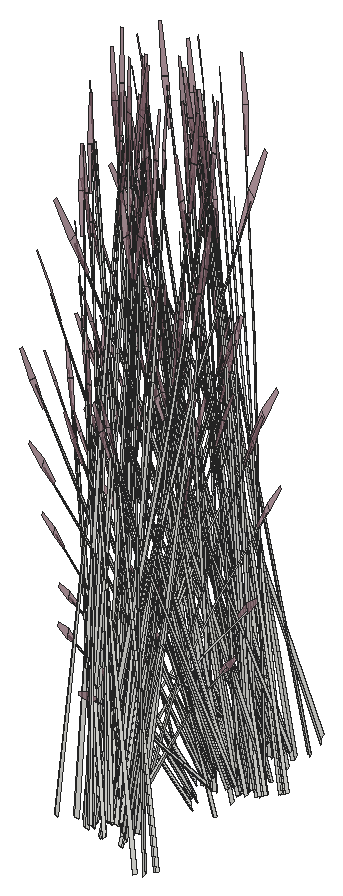
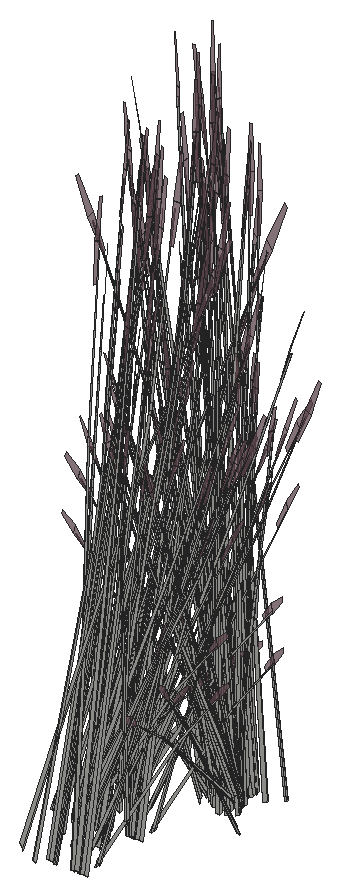
# SketchUp Ruby script. Lengths in inches.
U = 1.inch
M = Sketchup.active_model
def pt(a) = Geom::Point3d.new(a.map { |v| v * U })
def face(e, loops, mat)
  f = e.add_face(loops[0].map { |a| pt(a) })
  loops[1..].each { |l| e.add_face(l.map { |a| pt(a) }).erase! }
  f.material = f.back_material = mat if mat
  f
end
# faces: each face lists its corners as indices into pts; further lists are holes
def faces(e, pts, list, mat = nil) = list.each { |f| face(e, (f[0].is_a?(Array) ? f : [f]).map { |l| l.map { |i| pts[i] } }, mat) }
# xy, xz, yz: faces in a plane at the given z, y or x. An outline is a flat list of corners, or four numbers for a rectangle; further outlines are holes
def ring(l) = l.size == 4 ? [[l[0], l[1]], [l[2], l[1]], [l[2], l[3]], [l[0], l[3]]] : l.each_slice(2).to_a
def flat(e, list, mat, &to3) = list.each { |f| face(e, (f[0].is_a?(Array) ? f : [f]).map { |l| ring(l).map { |u, v| to3.(u, v) } }, mat) }
def xy(e, z, list, mat = nil) = flat(e, list, mat) { |x, y| [x, y, z] }
def xz(e, y, list, mat = nil) = flat(e, list, mat) { |x, z| [x, y, z] }
def yz(e, x, list, mat = nil) = flat(e, list, mat) { |y, z| [x, y, z] }
def lines(e, pts, list) = list.each { |a, b| e.add_line(pt(pts[a]), pt(pts[b])) }
# prism: a flat outline (further loops are holes) pulled along v
def prism(e, loops, v, mat = nil)
  f = face(e, loops, mat); d = Geom::Vector3d.new(v.map { |x| x * U })
  f.pushpull(f.normal.samedirection?(d) ? d.length : -d.length)
end
def box(e, o, s, mat = nil) = prism(e, [[o, [o[0] + s[0], o[1], o[2]], [o[0] + s[0], o[1] + s[1], o[2]], [o[0], o[1] + s[1], o[2]]]], [0, 0, s[2]], mat)
def at(x, y, z, deg = 0) = Geom::Transformation.translation(pt([x, y, z])) * Geom::Transformation.rotation(ORIGIN, Z_AXIS, deg.degrees)
def axes(o, x, y, z) = Geom::Transformation.new([*x, 0, *y, 0, *z, 0, *pt(o).to_a, 1])
def part(name) = M.definitions.add(name)
# library, detail: a bought-in or finely detailed component or shape, given as its bounding box
def library(name, o, s) = part(name).tap { |d| box(d.entities, o, s) }
def detail(e, o, s) = box(e.add_group.entities, o, s)
def put(e, d, t, mat = nil) = e.add_instance(d, t).tap { |i| i.material = mat if mat }
def group(e, t, mat = nil) = e.add_group.tap { |g| g.transformation = t; g.material = mat if mat }.entities
root = M.entities
M.materials.add("LightPink_Translucent").color = [144, 107, 117]
M.materials["LightPink_Translucent"].alpha = 0.75
c1 = part("blade")
p = [[2.15,0.21,22],[0,0.17,0],[0.09,0.45,0],[2.18,0.31,22],[2.29,0.31,22],[0.38,0.45,0],
  [2.48,0.24,33],[2.49,0.24,33],[2.48,0.22,33]]
faces(c1.entities,p,[[0,1,2,3],[4,5,2,3],[6,3,4,7],[8,0,3,6]])
c2 = part("seeds")
p = [[0.3,-0.1,1.38],[-0.01,-0.03,1.59],[-0.01,-0.03,0.03],[0.14,-0.07,-0.07],[0.29,-0.03,3],[0.15,0.01,3.11]]
faces(c2.entities,p,[[0,1,2,3],[1,0,4,5]],"LightPink_Translucent")
c3 = part("blade with seeds")
put(c3.entities,c1,at(0,0,0))
put(c3.entities,c2,axes([2.4,0.25,30.99],[1.5799,-0.05474,1.17369],[-0.12525,1.92788,0.29478],[-0.07173,-0.02425,1.56792]))
put(root,c3,axes([289.25,449.71,5.65],[0.78943,0.17416,-0.06488],[-0.24284,0.53604,-0.29416],[-0.12912,0.08139,0.97024]))
put(root,c3,axes([294.85,448.71,2.06],[-0.60257,0.49041,-0.62353],[-0.74854,-0.44469,-0.16365],[-0.24146,0.12234,1.37633]))
put(root,c3,axes([286.96,451.98,2.36],[-0.74176,0.59212,0.45755],[-0.88124,-0.52269,0.17955],[0.17882,-0.05909,1.58856]))
put(root,c3,axes([295.84,450.05,2.02],[-0.83726,0.32623,-0.49651],[-0.50045,-0.58498,0],[-0.19069,0.0743,1.57504]))
put(root,c3,axes([285.68,451.01,2.47],[-0.25843,0.64844,0.17642],[-0.9457,-0.1835,0.35086],[0.16336,-0.00316,1.60407]))
put(root,c3,axes([287.65,451.73,2.62],[0.17258,-0.58229,0.1448],[0.84319,0.10108,-0.41347],[0.15345,0.05979,1.26744]))
put(root,c3,axes([290.61,448.14,5.03],[0.82753,0.35977,-0.1216],[-0.47675,0.52101,-0.67495],[-0.2338,0.18111,1.02557]))
put(root,c3,axes([287.29,451.88,2.72],[-0.53742,-0.54764,0.44739],[0.81403,-0.38564,-0.21531],[0.17391,0.06776,1.43643]))
put(root,c3,axes([291.02,448.57,4.68],[0.22982,0.59576,-0.51099],[-0.87033,0.10422,-0.3958],[-0.24941,0.16002,0.97773]))
put(root,c3,axes([292.07,449.26,5.05],[0.60531,-0.34352,0.35414],[0.573,0.39225,-0.4572],[-0.08718,0.19929,0.87481]))
put(root,c3,axes([287.57,451.92,2.67],[0.90324,-0.43318,-0.29095],[0.60064,0.61207,-0.50002],[0.22285,0.06216,1.59708]))
put(root,c3,axes([296.125,447.36,2.84],[-0.02444,-0.61432,1.41272],[1.10603,0.15924,0.59816],[-0.26159,0.33615,1.3335]))
put(root,c3,axes([291.52,449.57,4.73],[-0.73517,-0.0304,0.0643],[0.02016,-0.45906,0.50621],[-0.07693,0.17585,0.77189]))
put(root,c3,axes([291.75,449.61,4.73],[-0.63704,-0.44518,0.48003],[0.67652,-0.38394,0.3958],[-0.11751,0.20886,0.9933]))
put(root,c3,axes([288.25,452.625,2.21],[1.00089,0,0],[0,0.67548,0],[0,0,1.78407]))
put(root,c3,axes([288.54,451.04,2.47],[-0.96132,0.17317,0.17642],[-0.23737,-0.64447,0.35086],[0.08574,0.0939,1.60407]))
put(root,c3,axes([289.61,451.01,2.03],[0.21015,0.56852,-0.30978],[-0.83462,0.16144,0.30978],[0.16826,0.06556,1.38974]))
put(root,c3,axes([287.93,452.28,2.38],[-1.13071,-0.13747,0.49198],[0.23011,-0.77639,0.19306],[0.16524,0.07497,1.70813]))
put(root,c3,axes([287.03,454.2,2.2],[-0.29189,-0.56252,0],[0.83351,-0.19699,0],[0,0,1.54371]))
put(root,c3,axes([291.56,448.48,3.875],[0.16657,-0.22426,1.71376],[0.69879,0.4641,0.13857],[-0.31524,0.28926,0.73262]))
put(root,c3,axes([288.12,454.12,2.18],[0.93921,-0.22138,-0.19198],[0.33003,0.6377,0.00008],[0.10367,-0.02447,1.73897]))
put(root,c3,axes([288.23,452.91,2.21],[0.62448,0.42144,0],[-0.62448,0.42144,0],[0,0,1.69266]))
put(root,c3,axes([289.92,452.73,2.47],[-0.70288,-0.47526,0.17642],[0.70832,-0.46097,0.35086],[-0.07763,0.09706,1.60407]))
put(root,c3,axes([291.75,449.74,4.53],[-0.60531,0.34352,-0.35414],[-0.573,-0.39225,0.4572],[-0.08718,0.19929,0.87481]))
put(root,c3,axes([289.66,449.64,4.72],[-0.02224,0.12912,1.74944],[0.63107,0.44917,-0.27667],[-0.16521,0.21241,0.14031]))
put(root,c3,axes([291.68,449.35,5.4],[0.98321,0.03233,-0.13498],[-0.02687,0.61208,-0.74919],[-0.0683,0.23574,1.13838]))
put(root,c3,axes([292.52,459.42,3.875],[0.2045,0.20949,1.71376],[-0.94495,0.17636,0.13857],[-0.21357,-0.32887,0.73262]))
put(root,c3,axes([292.14,451.08,2.77],[-0.02315,-0.38796,1.1486],[0.57853,0.27671,0.84392],[-0.11378,0.18492,0.25299]))
put(root,c3,axes([294.08,458.03,4.72],[-0.13683,-0.09148,1.74944],[-0.91315,0.058,-0.27667],[-0.14574,-0.2188,0.14031]))
put(root,c3,axes([288.22,452.42,2.72],[0.43405,-0.58792,0.44739],[0.90188,0.28295,-0.21531],[0,0.13553,1.43643]))
put(root,c3,axes([295.04,459.58,4.98],[-0.42698,-0.53052,-0.71045],[0.87893,-0.29566,0.08574],[-0.09984,-0.25633,1.00501]))
put(root,c3,axes([292.27,458.87,2.59],[-0.05417,0.21344,1.43002],[-0.79196,0.17867,-0.30754],[-0.18512,-0.27588,0.61141]))
put(root,c3,axes([288.06,452.76,2.29],[0,0.75458,-0.05637],[-1.11865,0,0],[0,0.02371,1.79368]))
put(root,c3,axes([288.14,452.22,2.21],[0.53742,0.54764,-0.44739],[-0.81403,0.38564,0.21531],[0.17391,0.06776,1.43643]))
put(root,c3,axes([292.35,449.58,5],[0.64041,0.4384,-0.5672],[-0.67652,0.38394,-0.43934],[-0.09744,0.22274,1.08528]))
put(root,c3,axes([291.66,450.24,2.82],[0.8127,-0.11554,0.06507],[0.18684,0.46549,-0.86304],[-0.05152,0.23564,0.7736]))
put(root,c3,axes([290.5,452.75,2.48],[0,-0.65246,0.49651],[1.00089,0,0],[0,0.1486,1.57504]))
put(root,c3,axes([287.99,453.24,2.72],[0.97146,-0.04028,0.44739],[0.08785,0.66859,-0.21531],[-0.17391,0.06776,1.43643]))
put(root,c3,axes([288.6,452.56,2.62],[0.83351,-0.19028,0.1448],[0.29189,0.54335,-0.41347],[0,0.11958,1.26744]))
put(root,c3,axes([292.15,449.38,5.34],[-0.02328,0.60353,-0.7886],[-0.98022,-0.04053,0.09517],[-0.10344,0.25568,1.11556]))
put(root,c3,axes([289.59,450.96,4.71],[0.10149,-0.03939,1.77383],[0.83886,0.26202,-0.16761],[-0.01971,0.21816,0.31391]))
put(root,c3,axes([287.85,454.46,2.2],[0.90188,0.29293,0],[-0.43405,0.60866,0],[0,0,1.74954]))
put(root,c3,axes([294.72,459.47,4.68],[-0.87941,-0.16356,-0.51099],[0.30143,-0.56078,-0.3958],[-0.08064,-0.22578,0.97773]))
put(root,c3,axes([293.08,448.95,3.875],[-0.0219,-0.25042,1.71376],[0.94901,0.16613,0.13857],[-0.0587,0.35688,0.73262]))
put(root,c3,axes([293.15,457.73,4.71],[-0.01669,0.07821,1.77383],[-0.82314,0.28383,-0.16761],[-0.24223,-0.14508,0.31391]))
put(root,c3,axes([292.97,459.12,5.09],[0.99656,-0.1677,0.53763],[0.17295,0.65785,0.4433],[-0.23438,-0.19388,1.11249]))
put(root,c3,axes([291.46,450.73,2.59],[0.28231,-0.10293,1.43002],[0.69701,0.31035,-0.30754],[-0.20746,0.26854,0.61141]))
put(root,c3,axes([295.47,459.44,5.03],[-0.87543,0.30377,-0.1216],[-0.4302,-0.53915,-0.67495],[-0.1155,-0.2272,1.02557]))
put(root,c3,axes([291.99,458.52,2.77],[0.46666,0.22709,1.1486],[-0.67962,0.13651,0.84392],[-0.14541,-0.17452,0.25299]))
put(root,c3,axes([288.71,454.73,2.48],[0.83726,-0.32623,0.49651],[0.50045,0.58498,0],[-0.19069,0.0743,1.57504]))
put(root,c3,axes([293.12,459.73,4.98],[-0.76283,-0.31537,-0.71045],[0.54213,-0.55263,0.08574],[-0.27638,-0.1883,1.00501]))
put(root,c3,axes([292.85,459.31,4.53],[-0.13817,-0.52554,-0.35414],[0.78985,-0.13877,0.4572],[-0.21215,-0.1506,0.87481]))
put(root,c3,axes([287.52,454.22,2.29],[0.38895,0.74956,-0.06012],[-1.11135,0.26265,0],[0.01358,0.02618,1.72173]))
put(root,c3,axes([291.18,452.86,2.375],[1.11865,0,0],[0,0.72922,-0.51607],[0,0.16609,1.63711]))
put(root,c3,axes([290.73,453.24,2.2],[-1.1181,-0.00522,-0.04976],[0,-0.72922,0.49943],[-0.03514,0.166,1.58352]))
put(root,c3,axes([288.32,452.6,2.67],[1.00749,0.31132,-0.29095],[-0.48511,0.65709,-0.50002],[0.03166,0.16133,1.59708]))
put(root,c3,axes([290.5,453.34,2.03],[-0.62448,0.40708,-0.30978],[-0.62448,-0.40708,0.30978],[0,0.13112,1.38974]))
put(root,c3,axes([291.83,450.23,3.36],[0.01966,-0.33682,1.54345],[0.88405,0.17791,0.21329],[-0.0766,0.35897,0.72882]))
put(root,c3,axes([293.2,459.26,4.73],[0.4066,-0.41448,0.0643],[0.57901,0.24131,0.50621],[-0.18719,-0.13288,0.77189]))
put(root,c3,axes([291.62,459.21,1.49],[-0.08666,0.08595,1.76342],[-0.87574,0.18531,-0.26939],[-0.21156,-0.16858,0.30037]))
put(root,c3,axes([288.21,453.09,2.21],[-0.43405,0.58792,-0.44739],[-0.90188,-0.28295,0.21531],[0,0.13553,1.43643]))
put(root,c3,axes([293.07,461.57,2.1],[-0.36739,-0.66907,-0.69835],[1.05831,-0.24096,-0.18329],[-0.04061,-0.22656,1.54149]))
put(root,c3,axes([292.76,459.74,4.68],[-0.88277,0.1551,-0.51099],[-0.15442,-0.58737,-0.3958],[-0.23711,-0.16832,0.97773]))
put(root,c3,axes([293.38,459.22,5.43],[-0.59706,0.6255,-0.13619],[-0.86465,-0.36036,-0.75594],[-0.30056,-0.17672,1.14864]))
put(root,c3,axes([287.96,454.97,5.05],[-0.13817,-0.52554,0.35414],[0.78985,-0.13877,-0.4572],[0.21215,0.1506,0.87481]))
put(root,c3,axes([288.23,454.78,2.33],[1.11998,0.21207,0.30756],[-0.2802,0.75803,-0.36492],[-0.18537,0.09487,1.64885]))
put(root,c3,axes([290.93,453.36,2.02],[0,0.65246,-0.49651],[-1.00089,0,0],[0,0.1486,1.57504]))
put(root,c3,axes([288.49,451.95,4.47],[-0.77304,-0.33901,1.38283],[0.81626,-0.52782,0.59665],[0.24941,0.31809,1.33663]))
put(root,c3,axes([294.15,458.86,2.13],[-0.61821,0.37431,-0.03893],[-0.56645,-0.40995,-0.17649],[-0.03988,-0.11616,0.58215]))
put(root,c3,axes([289.66,454.71,2.77],[-0.5037,-0.18761,1.1486],[0.6504,-0.19062,0.84392],[0.17543,0.16147,0.25299]))
put(root,c3,axes([294.94,463.29,3.33],[0.77308,0.2631,1.51261],[-0.75736,0.56681,0.59816],[-0.33924,-0.33594,1.26806]))
put(root,c3,axes([287.19,455.71,4.71],[0.00265,-0.07899,1.77383],[0.76665,-0.34851,-0.16761],[0.2663,0.12439,0.31391]))
put(root,c3,axes([293.32,459.74,5.05],[0.13817,0.52554,0.35414],[-0.78985,0.13877,-0.4572],[-0.21215,-0.1506,0.87481]))
put(root,c3,axes([288.72,453.27,2.09],[0.32803,0.59738,-0.69212],[-0.94492,0.21515,-0.18165],[0.03626,0.20229,1.52773]))
put(root,c3,axes([290.9,461.48,2.02],[0,-0.65246,-0.49651],[1.00089,0,0],[0,-0.1486,1.57504]))
put(root,c3,axes([286.07,455.06,5.05],[0.2697,-0.50175,0.35414],[0.78684,0.14635,-0.4572],[0.07215,0.20201,0.87481]))
put(root,c3,axes([289.74,455.5625,2.67],[-0.57368,-0.02046,1.0506],[0.37886,-0.43461,0.58006],[0.22663,0.15441,0.8241]))
put(root,c3,axes([288.09,455.45,4.73],[-0.4066,0.41448,0.0643],[-0.57901,-0.24131,0.50621],[0.18719,0.13288,0.77189]))
put(root,c3,axes([291.29,460.08,4.73],[0.04505,-0.49615,0.0643],[0.68022,0.0136,0.50621],[-0.26056,-0.05192,0.77189]))
put(root,c3,axes([287.13,456.85,5.65],[0.61821,-0.37431,-0.06488],[0.56645,0.40995,-0.29416],[0.03988,0.11616,0.97024]))
put(root,c3,axes([288.26,455.33,4.73],[-0.88979,0.14973,0.48003],[-0.15442,-0.58737,0.3958],[0.20926,0.17311,0.9933]))
put(root,c3,axes([291.33,461.49,2.03],[0.62448,-0.40708,-0.30978],[0.62448,0.40708,0.30978],[0,-0.13112,1.38974]))
put(root,c3,axes([291.08,459.54,2.13],[-0.25807,0.53277,-0.03893],[-0.79428,-0.16389,-0.17649],[-0.1206,-0.08714,0.58215]))
put(root,c3,axes([293.52,462.23,2.67],[-1.00749,-0.31132,-0.29095],[0.48511,-0.65709,-0.50002],[-0.03166,-0.16133,1.59708]))
put(root,c3,axes([290.65,461.97,2.375],[-1.11865,0,0],[0,-0.72922,-0.51607],[0,-0.16609,1.63711]))
put(root,c3,axes([287.87,454.51,2.59],[0.01579,-0.21629,1.43002],[0.75442,-0.24159,-0.30754],[0.23289,0.25887,0.61141]))
put(root,c3,axes([285.81,455.27,5.03],[0.87543,-0.30377,-0.1216],[0.4302,0.53915,-0.67495],[0.1155,0.2272,1.02557]))
put(root,c3,axes([285.97,455.38,1.49],[0.14478,-0.0355,1.76342],[0.8709,0.19542,-0.26939],[0.02547,0.22025,0.30037]))
put(root,c3,axes([291.52,461.78,2.33],[-0.83213,0.54855,0.30756],[-0.83263,-0.54278,-0.36492],[-0.02906,-0.15578,1.64885]))
put(root,c3,axes([286.5625,455.24,4.68],[0.87941,0.16356,-0.51099],[-0.30143,0.56078,-0.3958],[0.08064,0.22578,0.97773]))
put(root,c3,axes([287.0625,454.08,3.875],[-0.2045,-0.20949,1.71376],[0.94495,-0.17636,0.13857],[0.21357,0.32887,0.73262]))
put(root,c3,axes([293.77,462.92,2.4375],[0.23711,-0.77313,-0.23429],[1.12425,0.13477,0.51271],[-0.19645,-0.10677,1.5644]))
put(root,c3,axes([286.16,455.58,4.53],[-0.2697,0.50175,-0.35414],[-0.78684,-0.14635,0.4572],[0.07215,0.20201,0.87481]))
put(root,c3,axes([291.75,460.45,5.05],[0.50902,0.40851,0.35414],[-0.58122,0.38671,-0.4572],[-0.29531,-0.05884,0.87481]))
put(root,c3,axes([292.43,465.93,3.875],[0.2045,0.20949,1.71376],[-0.94495,0.17636,0.13857],[-0.21357,-0.32887,0.73262]))
put(root,c3,axes([291.33,462.08,2.48],[0,0.65246,0.49651],[-1.00089,0,0],[0,-0.1486,1.57504]))
put(root,c3,axes([293.99,464.54,4.72],[-0.13683,-0.09148,1.74944],[-0.91315,0.058,-0.27667],[-0.14574,-0.2188,0.14031]))
put(root,c3,axes([293.69,462.61,2.21],[-0.53742,-0.54764,-0.44739],[0.81403,-0.38564,0.21531],[-0.17391,-0.06776,1.43643]))
put(root,c3,axes([286.24,455.13,4.98],[0.42698,0.53052,-0.71045],[-0.87893,0.29566,0.08574],[0.09984,0.25633,1.00501]))
put(root,c3,axes([294.94,466.08,4.98],[-0.42698,-0.53052,-0.71045],[0.87893,-0.29566,0.08574],[-0.09984,-0.25633,1.00501]))
put(root,c3,axes([292.17,465.375,2.59],[-0.05417,0.21344,1.43002],[-0.79196,0.17867,-0.30754],[-0.18512,-0.27588,0.61141]))
put(root,c3,axes([293.61,462.41,2.72],[-0.43405,0.58792,0.44739],[-0.90188,-0.28295,-0.21531],[0,-0.13553,1.43643]))
put(root,c3,axes([285.6,456.47,4.72],[0.1134,0.10507,1.74944],[0.91515,0.04128,-0.27667],[0.09203,0.23172,0.14031]))
put(root,c3,axes([293.21,462.82,2.06],[-0.9306,-0.10697,-0.62353],[0.19638,-0.65984,-0.16365],[-0.27771,-0.07995,1.37633]))
put(root,c3,axes([294.625,465.98,4.68],[-0.87941,-0.16356,-0.51099],[0.30143,-0.56078,-0.3958],[-0.08064,-0.22578,0.97773]))
put(root,c3,axes([293.9,462.55,2.36],[1.13071,0.13747,0.45755],[-0.23011,0.77639,0.17955],[-0.16524,-0.07497,1.58856]))
put(root,c3,axes([292.22,463.82,2.03],[-0.21015,-0.56852,-0.30978],[0.83462,-0.16144,0.30978],[-0.16826,-0.06556,1.38974]))
put(root,c3,axes([293.05,464.24,4.71],[-0.01669,0.07821,1.77383],[-0.82314,0.28383,-0.16761],[-0.24223,-0.14508,0.31391]))
put(root,c3,axes([293.3,463.79,2.47],[0.96132,-0.17317,0.17642],[0.23737,0.64447,0.35086],[-0.08574,-0.0939,1.60407]))
put(root,c3,axes([292.87,465.625,5.09],[0.99656,-0.1677,0.53763],[0.17295,0.65785,0.4433],[-0.23438,-0.19388,1.11249]))
put(root,c3,axes([291.99,464.07,2.02],[-0.83726,-0.32623,-0.49651],[0.50045,-0.58498,0],[-0.19069,-0.0743,1.57504]))
put(root,c3,axes([295.375,465.95,5.03],[-0.87543,0.30377,-0.1216],[-0.4302,-0.53915,-0.67495],[-0.1155,-0.2272,1.02557]))
put(root,c3,axes([291.89,465.03,2.77],[0.46666,0.22709,1.1486],[-0.67962,0.13651,0.84392],[-0.14541,-0.17452,0.25299]))
put(root,c3,axes([293.02,466.23,4.98],[-0.76283,-0.31537,-0.71045],[0.54213,-0.55263,0.08574],[-0.27638,-0.1883,1.00501]))
put(root,c3,axes([294.27,462.92,2.67],[-0.90324,0.43318,-0.29095],[-0.60064,-0.61207,-0.50002],[-0.22285,-0.06216,1.59708]))
put(root,c3,axes([292.76,465.82,4.53],[-0.13817,-0.52554,-0.35414],[0.78985,-0.13877,0.4572],[-0.21215,-0.1506,0.87481]))
put(root,c3,axes([293.1,465.77,4.73],[0.4066,-0.41448,0.0643],[0.57901,0.24131,0.50621],[-0.18719,-0.13288,0.77189]))
put(root,c3,axes([291.52,465.71,1.49],[-0.08666,0.08595,1.76342],[-0.87574,0.18531,-0.26939],[-0.21156,-0.16858,0.30037]))
put(root,c3,axes([294.18,463.1,2.62],[-0.17258,0.58229,0.1448],[-0.84319,-0.10108,-0.41347],[-0.15345,-0.05979,1.26744]))
put(root,c3,axes([290.91,461.59,5.05],[0.74348,0.18202,0.35414],[-0.21685,0.53102,-0.4572],[-0.29933,0.04869,0.87481]))
put(root,c3,axes([292.97,468.08,2.1],[-0.36739,-0.66907,-0.69835],[1.05831,-0.24096,-0.18329],[-0.04061,-0.22656,1.54149]))
put(root,c3,axes([292.66,466.25,4.68],[-0.88277,0.1551,-0.51099],[-0.15442,-0.58737,-0.3958],[-0.23711,-0.16832,0.97773]))
put(root,c3,axes([295.28,463.11,2.46],[-0.87356,-0.52515,-0.25192],[0.73507,-0.5897,0.5513],[-0.23523,0.06143,1.68216]))
put(root,c3,axes([293.28,465.73,5.43],[-0.59706,0.6255,-0.13619],[-0.86465,-0.36036,-0.75594],[-0.30056,-0.17672,1.14864]))
put(root,c3,axes([292.98,464.12,2.48],[0.83726,0.32623,0.49651],[-0.50045,0.58498,0],[-0.19069,-0.0743,1.57504]))
put(root,c3,axes([294.05,465.36,2.13],[-0.61821,0.37431,-0.03893],[-0.56645,-0.40995,-0.17649],[-0.03988,-0.11616,0.58215]))
put(root,c3,axes([292.5,464.46,2.375],[-0.55932,0.6538,0],[-0.93577,-0.36461,-0.51607],[-0.21313,-0.08304,1.63711]))
put(root,c3,axes([294.84,463,2.21],[-0.97146,0.04028,-0.44739],[-0.08785,-0.66859,0.21531],[-0.17391,0.06776,1.43643]))
put(root,c3,axes([294.85,469.8,3.33],[0.77308,0.2631,1.51261],[-0.75736,0.56681,0.59816],[-0.33924,-0.33594,1.26806]))
put(root,c3,axes([293.22,466.25,5.05],[0.13817,0.52554,0.35414],[-0.78985,0.13877,-0.4572],[-0.21215,-0.1506,0.87481]))
put(root,c3,axes([290.8,467.98,2.02],[0,-0.65246,-0.49651],[1.00089,0,0],[0,-0.1486,1.57504]))
put(root,c3,axes([295.92,464.55,2.19],[-0.55235,-0.65609,-0.05142],[0.93577,-0.36461,0.51607],[-0.23059,0.06247,1.6363]))
put(root,c3,axes([291.1875,466.58,4.73],[0.04505,-0.49615,0.0643],[0.68022,0.0136,0.50621],[-0.26056,-0.05192,0.77189]))
put(root,c3,axes([291.23,468,2.03],[0.62448,-0.40708,-0.30978],[0.62448,0.40708,0.30978],[0,-0.13112,1.38974]))
put(root,c3,axes([290.98,466.05,2.13],[-0.25807,0.53277,-0.03893],[-0.79428,-0.16389,-0.17649],[-0.1206,-0.08714,0.58215]))
put(root,c3,axes([293.42,468.74,2.67],[-1.00749,-0.31132,-0.29095],[0.48511,-0.65709,-0.50002],[-0.03166,-0.16133,1.59708]))
put(root,c3,axes([295.66,464.47,2.03],[-0.83462,-0.16144,-0.30978],[0.21015,-0.56852,0.30978],[-0.16826,0.06556,1.38974]))
put(root,c3,axes([290.55,468.48,2.375],[-1.11865,0,0],[0,-0.72922,-0.51607],[0,-0.16609,1.63711]))
put(root,c3,axes([291.03,462.87,5.05],[0.77872,-0.09325,0.35414],[0.20563,0.53305,-0.4572],[-0.22316,0.14318,0.87481]))
put(root,c3,axes([295.52,462.82,2.67],[0.10425,0.7445,-0.29095],[-1.08575,0.04502,-0.50002],[-0.19119,0.09917,1.59708]))
put(root,c3,axes([291.42,468.29,2.33],[-0.83213,0.54855,0.30756],[-0.83263,-0.54278,-0.36492],[-0.02906,-0.15578,1.64885]))
put(root,c3,axes([289.27,464.38,5.65],[0.78943,0.17416,-0.06488],[-0.24284,0.53604,-0.29416],[-0.12912,0.08139,0.97024]))
put(root,c3,axes([294.87,463.39,2.06],[-0.60257,0.49041,-0.62353],[-0.74854,-0.44469,-0.16365],[-0.24146,0.12234,1.37633]))
put(root,c3,axes([293.67,469.43,2.4375],[0.23711,-0.77313,-0.23429],[1.12425,0.13477,0.51271],[-0.19645,-0.10677,1.5644]))
put(root,c3,axes([295.86,464.73,2.02],[-0.83726,0.32623,-0.49651],[-0.50045,-0.58498,0],[-0.19069,0.0743,1.57504]))
